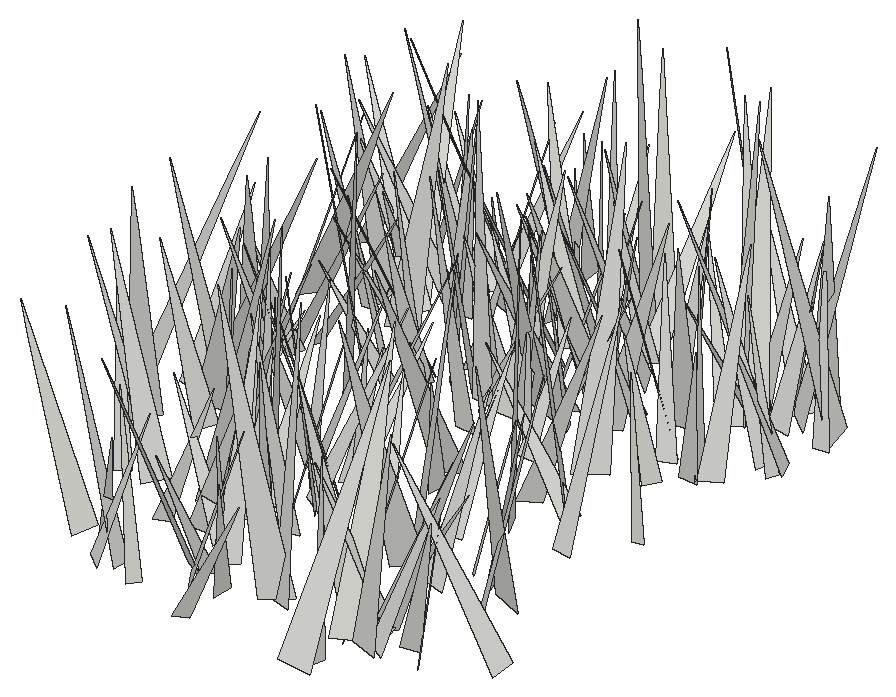
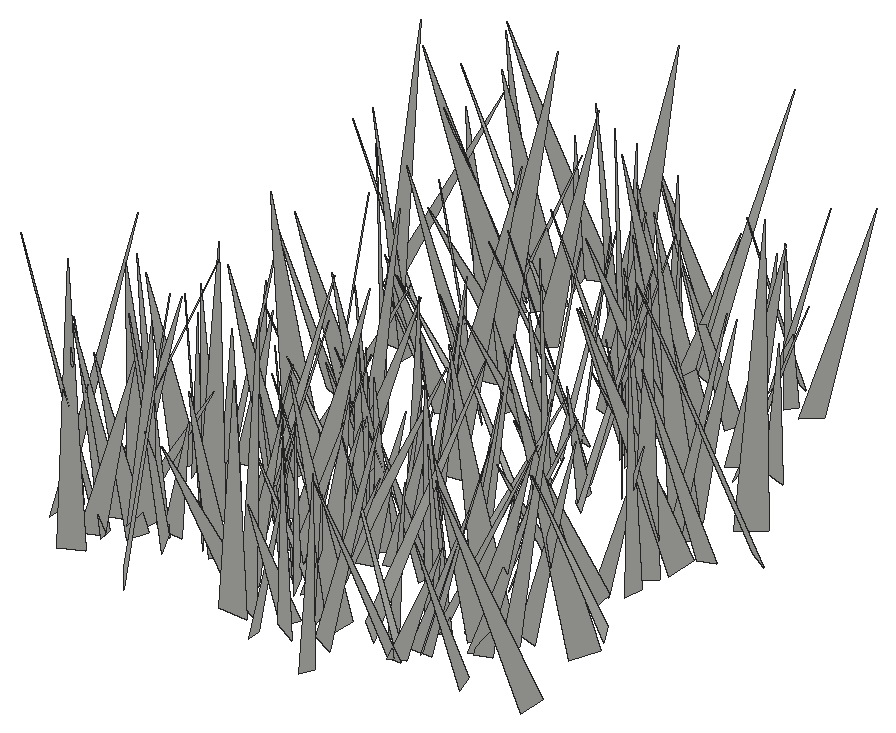
# SketchUp Ruby script. Lengths in inches.
U = 1.inch
M = Sketchup.active_model
def pt(a) = Geom::Point3d.new(a.map { |v| v * U })
def face(e, loops, mat)
  f = e.add_face(loops[0].map { |a| pt(a) })
  loops[1..].each { |l| e.add_face(l.map { |a| pt(a) }).erase! }
  f.material = f.back_material = mat if mat
  f
end
# faces: each face lists its corners as indices into pts; further lists are holes
def faces(e, pts, list, mat = nil) = list.each { |f| face(e, (f[0].is_a?(Array) ? f : [f]).map { |l| l.map { |i| pts[i] } }, mat) }
# xy, xz, yz: faces in a plane at the given z, y or x. An outline is a flat list of corners, or four numbers for a rectangle; further outlines are holes
def ring(l) = l.size == 4 ? [[l[0], l[1]], [l[2], l[1]], [l[2], l[3]], [l[0], l[3]]] : l.each_slice(2).to_a
def flat(e, list, mat, &to3) = list.each { |f| face(e, (f[0].is_a?(Array) ? f : [f]).map { |l| ring(l).map { |u, v| to3.(u, v) } }, mat) }
def xy(e, z, list, mat = nil) = flat(e, list, mat) { |x, y| [x, y, z] }
def xz(e, y, list, mat = nil) = flat(e, list, mat) { |x, z| [x, y, z] }
def yz(e, x, list, mat = nil) = flat(e, list, mat) { |y, z| [x, y, z] }
def lines(e, pts, list) = list.each { |a, b| e.add_line(pt(pts[a]), pt(pts[b])) }
# prism: a flat outline (further loops are holes) pulled along v
def prism(e, loops, v, mat = nil)
  f = face(e, loops, mat); d = Geom::Vector3d.new(v.map { |x| x * U })
  f.pushpull(f.normal.samedirection?(d) ? d.length : -d.length)
end
def box(e, o, s, mat = nil) = prism(e, [[o, [o[0] + s[0], o[1], o[2]], [o[0] + s[0], o[1] + s[1], o[2]], [o[0], o[1] + s[1], o[2]]]], [0, 0, s[2]], mat)
def at(x, y, z, deg = 0) = Geom::Transformation.translation(pt([x, y, z])) * Geom::Transformation.rotation(ORIGIN, Z_AXIS, deg.degrees)
def axes(o, x, y, z) = Geom::Transformation.new([*x, 0, *y, 0, *z, 0, *pt(o).to_a, 1])
def part(name) = M.definitions.add(name)
# library, detail: a bought-in or finely detailed component or shape, given as its bounding box
def library(name, o, s) = part(name).tap { |d| box(d.entities, o, s) }
def detail(e, o, s) = box(e.add_group.entities, o, s)
def put(e, d, t, mat = nil) = e.add_instance(d, t).tap { |i| i.material = mat if mat }
def group(e, t, mat = nil) = e.add_group.tap { |g| g.transformation = t; g.material = mat if mat }.entities
root = M.entities
c1 = part("fur_instance\#9")
p = [[0.8125,0,1.79],[0.67,-0.02,1.48],[0,-0.11,0],[0,0.11,0]]
faces(c1.entities,p,[[0,1,2,3]])
put(root,c1,axes([476.24,187.77,-21.66],[4.4489,2.71988,0.66857],[2.4928,-4.41728,1.38241],[-1.27698,0.85286,5.02786]))
put(root,c1,axes([474.66,195.15,-21.66],[5.89255,-1.31891,0.46121],[-1.38894,-5.74659,1.31223],[-0.15186,1.38261,5.89404]))
put(root,c1,axes([475.08,177.99,-21.66],[4.54632,6.46757,0.61256],[6.48609,-4.47646,-0.87508],[0.36794,-1.0028,7.85702]))
put(root,c1,axes([478.71,179.93,-21.66],[-6.26748,-0.84521,1.62615],[-0.68504,6.45447,0.7145],[1.69984,-0.51518,6.28372]))
put(root,c1,axes([476.84,179.58,-21.66],[0.12132,5.40428,1.16344],[5.42728,0.10479,-1.05269],[1.05091,-1.16504,5.30215]))
put(root,c1,axes([478.76,190.43,-21.66],[-1.01611,-5.1437,1.43202],[-5.3112,0.8243,-0.80778],[-0.54728,1.55038,5.1805]))
put(root,c1,axes([477.09,176.02,-21.66],[5.45655,-4.97036,1.37233],[-4.9464,-5.60993,-0.6508],[-1.45634,0.43117,7.35221]))
put(root,c1,axes([478.71,191.72,-21.66],[-6.33484,-0.15602,2.15214],[0.09289,6.64883,0.75543],[2.15578,-0.74496,6.29157]))
put(root,c1,axes([479.32,171.53,-21.66],[-0.14147,5.00237,0.6936],[4.87308,-0.04695,1.33257],[-1.32587,-0.70632,4.82369]))
put(root,c1,axes([477.64,183.99,-21.66],[5.74214,0.07937,1.80023],[0.34922,-5.94743,-0.85168],[-1.76782,-0.91707,5.67918]))
put(root,c1,axes([478.67,185.1,-21.66],[2.63547,-2.52355,0.88422],[-2.24578,-2.7628,-1.19134],[-1.45143,-0.30736,3.44888]))
put(root,c1,axes([480.8125,172.24,-21.66],[-5.83458,-0.97839,0.23219],[-1.00024,5.78729,-0.74851],[0.10327,0.77686,5.8685]))
put(root,c1,axes([480.66,191.54,-21.66],[-3.78677,4.88862,0.77178],[4.90876,3.58599,1.37062],[-0.63111,-1.44081,6.0299]))
put(root,c1,axes([475.72,189.9375,-21.66],[6.5822,-3.48627,0.04021],[-3.46978,-6.5418,0.80411],[0.34104,0.72931,7.40492]))
put(root,c1,axes([479.73,192.85,-21.66],[-4.18916,1.41328,1.44955],[1.84035,4.04661,1.3732],[0.84361,-1.80976,4.20247]))
put(root,c1,axes([478.39,195.45,-21.66],[4.03699,1.00135,1.00845],[0.75439,-4.0837,1.03503],[-1.2044,0.79854,4.02849]))
put(root,c1,axes([479.79,177.1,-21.66],[3.58153,-3.37168,2.12142],[-3.21603,-4.13077,-1.13573],[-2.3507,0.51427,4.78599]))
put(root,c1,axes([477.99,182.7,-21.66],[6.15158,-3.29467,0.71793],[-3.15743,-6.15236,-1.17953],[-1.18361,-0.7112,6.87789]))
put(root,c1,axes([480.25,191.67,-21.66],[-4.33285,5.33033,0.39838],[5.19442,4.31986,-1.30443],[1.26061,0.52067,6.74422]))
put(root,c1,axes([479.34,192.875,-21.66],[2.09335,-3.21544,0.11512],[-3.16402,-2.08217,-0.6229],[-0.58423,-0.24481,3.78592]))
put(root,c1,axes([477.34,180.83,-21.66],[6.84085,-1.05323,0.60817],[-1.14548,-6.7472,1.19982],[-0.40871,1.28156,6.81667]))
put(root,c1,axes([481.98,193.72,-21.66],[-6.45817,-1.9042,0.82118],[-2.02073,6.38203,-1.093],[0.4658,1.28531,6.64374]))
put(root,c1,axes([481.15,171.73,-21.66],[-4.7653,3.97573,1.88545],[4.327,4.73874,0.94381],[0.79899,-1.95123,6.13381]))
put(root,c1,axes([478.27,185.5,-21.66],[5.14686,-0.10254,0.48257],[-0.21946,-5.00543,1.27711],[-0.44184,1.29176,4.98695]))
put(root,c1,axes([481.48,166.06,-21.66],[-5.50696,2.25656,1.40845],[2.52369,5.45565,1.12666],[0.84072,-1.59571,5.84374]))
put(root,c1,axes([482.23,192.55,-21.66],[-5.87087,-0.65311,0.1721],[-0.62527,5.82501,0.77566],[0.25536,-0.75237,5.85594]))
put(root,c1,axes([481.77,194.43,-21.66],[-2.38269,3.95567,1.05235],[4.03891,2.07425,1.34786],[-0.66484,-1.57548,4.41677]))
put(root,c1,axes([482.22,195.6,-21.66],[-3.14834,2.92622,0.07201],[2.87738,3.07451,0.86494],[-0.53726,-0.68166,4.21031]))
put(root,c1,axes([478.875,186.36,-21.66],[4.0967,-0.1052,0.02727],[-0.10864,-3.93802,1.12914],[0.00278,1.12946,3.93942]))
put(root,c1,axes([482.51,186.8,-21.66],[-3.84784,-1.19504,0.32807],[-1.23606,3.62421,-1.29571],[-0.08892,1.33363,3.81512]))
put(root,c1,axes([481.8,189.2,-21.66],[-3.17916,-2.57933,0.00353],[-2.53731,3.12837,0.73174],[0.46373,-0.56605,4.02798]))
put(root,c1,axes([478.75,178.69,-21.66],[3.49272,-6.19271,0.17705],[-6.11252,-3.41157,1.25629],[1.00898,0.76914,6.99789]))
put(root,c1,axes([480.98,190.02,-21.66],[5.12672,-4.5376,2.59386],[-5.0883,-5.16347,1.02416],[-1.19461,2.5199,6.76936]))
put(root,c1,axes([482.89,191.59,-21.66],[-5.05417,-1.27819,2.14403],[-1.86511,5.15169,-1.32541],[1.65892,1.89778,5.04199]))
put(root,c1,axes([481.2,178.72,-21.66],[3.19088,3.17646,1.19509],[3.39239,-3.03309,-0.99593],[-0.09903,-1.55252,4.39087]))
put(root,c1,axes([484.76,187.57,-21.66],[-3.76268,-4.24685,0.11424],[-4.17448,3.66755,-1.15295],[-0.78896,0.84846,5.55555]))
put(root,c1,axes([484.8,164.57,-21.66],[-6.17227,-0.98801,0.5453],[-1.07692,6.06305,-1.2042],[0.3373,1.27815,6.13375]))
put(root,c1,axes([484.81,194.36,-21.66],[-4.99858,-6.00178,0.67378],[-6.03784,4.94565,-0.739],[-0.1407,0.9901,7.77567]))
put(root,c1,axes([481.07,176.93,-21.66],[1.22352,3.80068,0.33063],[3.61313,-1.04295,-1.38167],[1.22465,-0.72012,3.74608]))
put(root,c1,axes([484.16,185.24,-21.66],[-3.93279,-0.23592,0.50656],[-0.05149,3.7386,1.34138],[0.55643,-1.32147,3.70448]))
put(root,c1,axes([483.9375,176.93,-21.66],[2.37526,2.53476,1.46683],[2.25858,-2.78775,1.16004],[-1.86424,-0.14786,3.27432]))
put(root,c1,axes([482.27,192.54,-21.66],[2.19919,-5.46865,1.19281],[-5.58851,-2.07385,0.79564],[0.31218,1.39943,5.84033]))
put(root,c1,axes([482.7,183.87,-21.66],[6.58164,2.52237,2.667],[2.99732,-6.85363,-0.91486],[-2.11926,-1.85972,6.9888]))
put(root,c1,axes([485.0625,182.67,-21.66],[-5.96506,-5.04673,2.13711],[-5.35643,6.03696,-0.69462],[1.15994,1.92465,7.7826]))
put(root,c1,axes([484.43,172.75,-21.66],[-4.83197,-1.5354,1.95575],[-2.0901,4.8234,-1.3772],[1.34681,1.9768,4.87942]))
put(root,c1,axes([482.3,195.72,-21.66],[1.86244,4.7215,0.55373],[4.68693,-1.72429,-1.06173],[0.79484,-0.89561,4.96326]))
put(root,c1,axes([482.78,165.92,-21.66],[3.65052,-1.24636,0.3015],[-1.17659,-3.61738,-0.70767],[-0.50984,-0.576,3.79195]))
put(root,c1,axes([484.67,179.25,-21.66],[-4.07639,-4.57708,0.71562],[-4.52519,4.13816,0.69067],[0.99219,0.06853,6.09012]))
put(root,c1,axes([485.39,177.82,-21.66],[-6.52757,-2.25287,1.08541],[-2.07972,6.57544,1.14066],[1.38863,-0.74224,6.81054]))
put(root,c1,axes([483.55,194.23,-21.66],[-0.85908,-3.57953,0.71794],[-3.54097,0.99653,0.73143],[0.88884,0.51028,3.60778]))
put(root,c1,axes([482.57,194.99,-21.66],[4.81991,2.46867,0.79438],[2.57067,-4.76928,-0.77622],[-0.3421,-1.05666,5.35942]))
put(root,c1,axes([485.87,185.33,-21.66],[-5.27526,-0.92635,0.94955],[-1.13263,5.17215,-1.24665],[0.69057,1.40673,5.20887]))
put(root,c1,axes([484.89,178.5,-21.66],[-3.85021,0.78609,0.9669],[0.45373,3.80886,-1.28983],[1.16059,1.11875,3.71193]))
put(root,c1,axes([485.46,174.22,-21.66],[-5.53054,0.45224,1.5037],[0.10523,5.59989,-1.29715],[1.5667,1.22031,5.39525]))
put(root,c1,axes([485.76,196.62,-21.66],[-2.42816,-5.42807,1.43938],[-5.61543,2.33238,-0.67728],[-0.05217,1.5899,5.90772]))
put(root,c1,axes([486.3125,163.6,-21.66],[-4.58917,0.765,0.19448],[0.68534,4.43094,-1.25723],[0.3916,1.21042,4.47941]))
put(root,c1,axes([483.6,164.08,-21.66],[2.51167,3.62255,0.80621],[3.69421,-2.34748,-0.96099],[0.35452,-1.20325,4.30208]))
put(root,c1,axes([483.6875,169.01,-21.66],[3.11489,-2.67244,0.85057],[-2.80172,-2.90834,1.1224],[0.12545,1.40269,3.94774]))
put(root,c1,axes([483.26,173.39,-21.66],[6.3266,0.04535,0.7535],[-0.10627,-6.24313,1.26797],[-0.74735,1.27161,6.1984]))
put(root,c1,axes([485.06,186.32,-21.66],[3.85472,-3.45884,0.89823],[-3.26491,-3.94586,-1.18314],[-1.45282,-0.30973,5.04209]))
put(root,c1,axes([483.9,172.14,-21.66],[7.6269,-0.50277,1.8471],[-0.68475,-7.80192,0.70374],[-1.78765,0.84341,7.61099]))
put(root,c1,axes([484.76,199.0625,-21.66],[4.55576,-0.64185,1.19418],[-0.37344,-4.61891,-1.05794],[-1.3033,-0.92017,4.47746]))
put(root,c1,axes([487.13,169.12,-21.66],[-3.1283,2.85302,0.75954],[2.94685,2.94951,1.058],[-0.18092,-1.28978,4.09959]))
put(root,c1,axes([486.23,171.21,-21.66],[-5.56085,2.56326,1.5764],[2.25423,5.74256,-1.38556],[1.99343,0.65656,5.96435]))
put(root,c1,axes([486.22,187.08,-21.66],[4.10758,4.73433,2.04961],[4.7509,-4.49256,0.85604],[-2.01089,-0.9434,6.20913]))
put(root,c1,axes([486.87,187.87,-21.66],[-4.89402,-3.33819,1.83703],[-3.30827,5.20635,0.64726],[1.89038,0.46913,5.88863]))
put(root,c1,axes([488.79,191.91,-21.66],[-3.68425,-5.36529,0.32526],[-5.32374,3.58793,-1.11818],[-0.74155,0.8979,6.41168]))
put(root,c1,axes([486.41,173.12,-21.66],[-2.91269,3.59929,0.76549],[3.33369,2.99435,-1.39463],[1.55801,0.3218,4.41516]))
put(root,c1,axes([486.15,172.15,-21.66],[-1.6675,3.7386,1.84502],[3.94069,2.06209,-0.61692],[1.36097,-1.39013,4.04687]))
put(root,c1,axes([485.87,188.88,-21.66],[3.36091,-1.13304,0.9234],[-1.35023,-3.29337,0.87337],[-0.55977,1.1411,3.43755]))
put(root,c1,axes([487.35,194.96,-21.66],[-3.69275,-0.52533,1.17947],[-0.76187,3.77166,-0.70545],[1.04243,0.89562,3.66261]))
put(root,c1,axes([487.93,193.75,-21.66],[-0.66847,-3.61729,0.84651],[-3.58891,0.40659,-1.09666],[-0.95975,0.99906,3.51127]))
put(root,c1,axes([488.29,193.41,-21.66],[-2.02202,5.92033,1.45384],[6.05855,1.78151,1.17164],[-0.67672,-1.74024,6.14542]))
put(root,c1,axes([487.82,196.84,-21.66],[1.64216,5.46326,1.64146],[5.44457,-2.0108,1.24565],[-1.70244,-1.16093,5.56707]))
put(root,c1,axes([486.04,194.98,-21.66],[6.43486,-0.85229,1.84553],[-1.08084,-6.62327,0.70985],[-1.72168,0.97247,6.45212]))
put(root,c1,axes([486.18,173.95,-21.66],[7.03768,2.72348,2.80411],[3.28727,-7.24831,-1.21043],[-2.11523,-2.20318,7.44856]))
put(root,c1,axes([487.78,166.26,-21.66],[-3.38776,-6.42257,0.32475],[-6.36234,3.40084,0.88702],[0.93573,-0.12917,7.20691]))
put(root,c1,axes([487.82,188.95,-21.66],[1.8485,-3.49978,1.33816],[-3.45042,-2.17169,-0.91344],[-1.46071,0.70098,3.8511]))
put(root,c1,axes([485.56,169.36,-21.66],[2.4486,-4.30122,0.69777],[-4.269,-2.2075,1.37318],[0.8735,1.26866,4.75506]))
put(root,c1,axes([488.29,186.8,-21.66],[1.87849,6.8023,2.53671],[7.02619,-2.36292,1.13321],[-1.82724,-2.09291,6.96533]))
put(root,c1,axes([488.79,187.26,-21.66],[-4.99068,-1.45127,1.21381],[-1.71677,4.91279,-1.18474],[0.79513,1.49823,5.06058]))
put(root,c1,axes([488.5625,174.17,-21.66],[3.89411,3.28531,3.07479],[3.51498,-4.75969,0.63397],[-2.80935,-1.40135,5.05524]))
put(root,c1,axes([489.1,193.22,-21.66],[-4.79619,2.23097,0.90337],[2.34699,4.78153,0.65218],[0.53379,-0.97799,5.24932]))
put(root,c1,axes([488.39,166.53,-21.66],[0.67909,-3.62862,0.46379],[-3.53581,-0.77205,-0.86319],[-0.93808,0.2832,3.58928]))
put(root,c1,axes([488.13,196.03,-21.66],[-2.89622,3.26829,0.45856],[3.08153,2.89643,-1.18106],[1.18158,0.4572,4.20415]))
put(root,c1,axes([489.01,171.71,-21.66],[-0.52973,-5.32119,2.08202],[-5.65742,0.19488,-0.94137],[-0.8022,2.1395,5.26399]))
put(root,c1,axes([488.3,176.08,-21.66],[-3.60567,-4.25836,0.82426],[-4.10665,3.69659,1.13335],[1.39586,-0.12438,5.46351]))
put(root,c1,axes([485.75,181.77,-21.66],[5.05169,2.87341,0.23488],[2.86098,-4.93803,-1.1233],[0.35552,-1.09113,5.70213]))
put(root,c1,axes([488.9,189.55,-21.66],[-2.91756,2.69263,1.56889],[3.08399,2.80363,0.92331],[0.448,-1.76443,3.86133]))
put(root,c1,axes([488.51,167.69,-21.66],[-5.11212,3.73872,1.49873],[3.53116,5.32488,-1.23875],[1.93782,0.15985,6.21106]))
put(root,c1,axes([487.84,168.29,-21.66],[3.54062,0.10617,1.20258],[0.38468,-3.63127,-0.812],[-1.14433,-0.89222,3.44788]))
put(root,c1,axes([488.78,197.92,-21.66],[-4.40075,-1.21691,1.44212],[-0.98766,4.60363,0.87078],[1.60783,-0.50284,4.4821]))
put(root,c1,axes([489.28,184.29,-21.66],[1.25077,5.74635,3.18749],[6.40163,-1.79789,0.7292],[-1.48314,-2.91412,5.83551]))
put(root,c1,axes([488.14,177.04,-21.66],[-2.24113,2.46388,1.48853],[2.36542,2.65133,-0.82724],[1.6405,-0.45695,3.22631]))
put(root,c1,axes([486.77,175.98,-21.66],[4.58071,3.98416,0.78034],[4.05613,-4.44078,-1.1369],[0.17387,-1.36793,5.96354]))
put(root,c1,axes([490.03,193.15,-21.66],[-4.76219,-1.42096,1.84075],[-1.91994,4.76946,-1.2853],[1.31199,1.82182,4.80058]))
put(root,c1,axes([489.7,175.6,-21.66],[-4.04138,0.55951,1.25439],[0.25517,4.13619,-1.02282],[1.34961,0.89343,3.94964]))
put(root,c1,axes([490.82,192.64,-21.66],[-2.4507,-4.58404,1.24543],[-4.71435,2.17524,-1.27033],[-0.58261,1.68089,5.0404]))
put(root,c1,axes([490.36,196.36,-21.66],[-3.60643,-6.53276,3.39182],[-7.2869,3.70246,-0.61691],[1.0404,3.28673,7.43658]))
put(root,c1,axes([488.8,176.6,-21.66],[-0.26739,4.57604,0.32256],[4.40279,0.34673,-1.26925],[1.2883,-0.2352,4.40462]))
put(root,c1,axes([490.78,196.97,-21.66],[-0.82841,6.75025,1.93378],[7.00258,0.65031,0.72978],[-0.51887,-2.00072,6.76162]))
put(root,c1,axes([488.21,174.43,-21.66],[2.55836,5.15566,0.46861],[5.11042,-2.43162,-1.14739],[0.82709,-0.92305,5.63999]))
put(root,c1,axes([488.95,188.11,-21.66],[1.24719,-3.91493,0.4967],[-3.8954,-1.13791,0.81231],[0.63182,0.71228,4.02769]))
put(root,c1,axes([488.31,165.21,-21.66],[4.57096,2.53062,0.74602],[2.63797,-4.36083,-1.37058],[0.04077,-1.55993,5.04174]))
put(root,c1,axes([489.68,169.35,-21.66],[-1.49561,-5.63035,1.67127],[-5.71638,1.79132,0.91926],[1.34798,1.34949,5.75262]))
put(root,c1,axes([489.92,192.4,-21.66],[3.50829,2.33455,0.59392],[2.17247,-3.51961,1.00185],[-1.04078,0.52272,4.09323]))
put(root,c1,axes([489.66,170.14,-21.66],[4.69636,2.95892,0.9191],[2.85112,-4.78039,0.82137],[-1.21287,0.21986,5.48965]))
put(root,c1,axes([489.66,189.04,-21.66],[-0.19463,-4.95849,1.24268],[-5.00803,0.4343,0.94858],[1.02496,1.18047,4.8708]))
put(root,c1,axes([488.2,186.69,-21.66],[4.34126,2.62004,0.01209],[2.52851,-4.18338,-1.34808],[0.68659,-1.1602,4.88813]))
put(root,c1,axes([490.1875,188.08,-21.66],[-1.33091,-4.34516,1.37723],[-4.35803,1.6335,0.94222],[1.33595,0.99989,4.44566]))
put(root,c1,axes([491.89,190.35,-21.66],[-4.72142,-2.258,0.83052],[-2.14472,4.77905,0.80066],[1.09019,-0.37724,5.17198]))
put(root,c1,axes([491.8125,188.625,-21.66],[0.91658,-6.09487,0.23316],[-5.96683,-0.94489,-1.24341],[-1.26442,0.04079,6.03668]))
put(root,c1,axes([490.07,165.45,-21.66],[3.94789,-1.4658,0.35037],[-1.34081,-3.86465,-1.06014],[-0.68816,-0.87925,4.0756]))
put(root,c1,axes([492.36,166.5625,-21.66],[2.49125,-7.31611,3.2771],[-7.62751,-3.2193,-1.38865],[-2.46697,2.5655,7.60286]))
put(root,c1,axes([489.58,191.08,-21.66],[4.36053,2.62617,0.62372],[2.69593,-4.29581,-0.7602],[-0.13318,-0.97427,5.03319]))
put(root,c1,axes([490.16,186.51,-21.66],[-1.02594,6.32348,2.52203],[6.58274,1.57191,-1.26344],[1.73626,-2.22313,6.28034]))
put(root,c1,axes([491.23,180.76,-21.66],[2.31085,-7.14722,0.11909],[-7.10013,-2.30949,-0.83147],[-0.82765,-0.14321,7.46535]))
put(root,c1,axes([491.9375,194.39,-21.66],[1.8151,-3.86013,1.55176],[-3.9232,-2.15155,-0.76319],[-1.38458,1.03602,4.19675]))
put(root,c1,axes([490.71,192.625,-21.66],[4.61711,2.95667,1.94744],[3.35791,-4.67134,-0.86895],[-1.12198,-1.8135,5.41336]))
put(root,c1,axes([492.01,190.66,-21.66],[1.78326,-6.33726,0.7797],[-6.26284,-1.89367,-1.06754],[-1.24322,0.44943,6.49625]))
put(root,c1,axes([490.88,187.85,-21.66],[-1.24529,-7.71146,0.7872],[-7.61167,1.36728,1.35282],[1.46589,0.54863,7.69333]))
put(root,c1,axes([492.83,187.4,-21.66],[-3.64875,-2.02244,1.121],[-2.25149,3.58457,-0.86132],[0.52696,1.3118,4.08188]))
put(root,c1,axes([491.42,195.37,-21.66],[-1.51981,5.35977,0.02073],[5.22969,1.48762,-1.21441],[1.17387,0.31183,5.43711]))
put(root,c1,axes([489.99,162.49,-21.66],[3.34433,-2.45993,0.06359],[-2.39384,-3.22746,1.0454],[0.56992,0.87868,4.01783]))
put(root,c1,axes([492.64,174.16,-21.66],[-3.06168,2.49465,0.02952],[2.42804,2.99025,-0.87237],[0.57338,0.65813,3.85176]))
put(root,c1,axes([490.96,186.12,-21.66],[-2.2184,-4.85625,2.50772],[-5.03427,2.86928,1.10295],[2.1279,1.72546,5.22379]))
put(root,c1,axes([492.61,184.6875,-21.66],[1.15906,3.62365,1.13013],[3.60388,-1.42153,0.86183],[-1.19166,-0.77453,3.7056]))
put(root,c1,axes([493.05,192.97,-21.66],[-5.52274,-3.05851,1.02558],[-2.84433,5.57616,1.31266],[1.52186,-0.67738,6.17511]))
put(root,c1,axes([490.95,192.83,-21.66],[4.30698,0.82715,0.77594],[0.97071,-4.26434,-0.84231],[-0.5865,-0.98365,4.30404]))
put(root,c1,axes([492.85,166.24,-21.66],[2.9733,6.47594,2.08154],[6.51847,-3.36189,1.14821],[-1.94427,-1.36785,7.03277]))
put(root,c1,axes([491.71,179.16,-21.66],[3.65469,-1.69105,0.3912],[-1.57801,-3.61693,-0.89287],[-0.72291,-0.65395,3.92673]))
put(root,c1,axes([493.05,183.98,-21.66],[-0.85161,3.55792,0.87868],[3.50079,1.05663,-0.88551],[1.08413,-0.61714,3.54963]))
put(root,c1,axes([493.64,175.32,-21.66],[4.42049,5.15695,1.86392],[5.12768,-4.73588,0.94203],[-1.94301,-0.76574,6.72662]))
put(root,c1,axes([494.09,191.12,-21.66],[-2.87377,-5.9267,0.11201],[-5.79461,2.83495,1.33509],[1.24935,-0.48389,6.44995]))
put(root,c1,axes([495.21,168.55,-21.66],[4.87258,-2.82126,2.84071],[-2.53321,-5.63755,-1.25383],[-3.10033,0.17232,5.48903]))
put(root,c1,axes([494.65,193.14,-21.66],[3.28542,-2.52777,1.83261],[-2.97263,-3.34603,0.71392],[-0.95477,1.71946,4.08337]))
put(root,c1,axes([495.21,172.72,-21.66],[3.52334,-7.25518,1.10129],[-7.15699,-3.66725,-1.26216],[-1.62106,0.42196,7.96608]))
put(root,c1,axes([493.16,185.2,-21.66],[4.26257,2.91433,0.00484],[2.86478,-4.18851,-0.95515],[0.53516,-0.79116,5.0745]))
put(root,c1,axes([496.79,197.47,-21.66],[-6.4254,-4.61842,2.37343],[-5.01235,6.50279,-0.91585],[1.35622,2.15235,7.85982]))
put(root,c1,axes([494.95,176.11,-21.66],[-1.9043,4.31856,1.08738],[4.14528,2.15112,-1.28374],[1.62757,-0.42591,4.54184]))
put(root,c1,axes([495.16,174.45,-21.66],[3.38702,2.66566,0.2184],[2.51461,-3.29384,1.20529],[-0.91115,0.81867,4.13823]))
put(root,c1,axes([496.16,188.73,-21.66],[-3.36385,-0.86607,1.07357],[-0.51946,3.41676,1.12873],[1.27781,-0.89095,3.28504]))
put(root,c1,axes([494.32,188.43,-21.66],[4.99795,-3.82327,1.26682],[-4.01963,-4.86241,1.18375],[-0.25457,1.71502,6.18026]))
put(root,c1,axes([496.3,184.66,-21.66],[5.95771,-4.00613,4.25574],[-5.13988,-6.48421,1.09155],[-2.78246,3.40011,7.09591]))
put(root,c1,axes([497.56,192.92,-21.66],[-1.2405,4.10694,0.41743],[4.03089,1.11105,1.04764],[-0.89058,-0.69186,4.16031]))
put(root,c1,axes([496.49,178.6875,-21.66],[6.19858,3.66698,3.16063],[3.75526,-6.8827,0.6206],[-3.05522,-1.01998,7.17523]))
put(root,c1,axes([498.41,180.68,-21.66],[-4.58076,1.47717,0.18742],[1.47131,4.39705,1.30451],[-0.22897,-1.29786,4.63288]))
put(root,c1,axes([497.93,180.97,-21.66],[-5.99226,-3.56649,1.99916],[-3.93709,5.99,-1.11487],[1.10264,2.00593,6.88361]))
put(root,c1,axes([495.87,192.83,-21.66],[4.89735,3.35239,2.18214],[3.80193,-4.97328,-0.89225],[-1.24321,-2.00306,5.86741]))
put(root,c1,axes([497.58,163.13,-21.66],[-4.70779,-0.34884,1.44292],[-0.70643,4.74641,-1.15738],[1.30563,1.3103,4.57662]))
put(root,c1,axes([498.45,167.41,-21.66],[-4.68733,-0.90911,0.30449],[-0.85582,4.65242,0.7161],[0.43216,-0.64711,4.72067]))
put(root,c1,axes([497.28,165.61,-21.66],[-5.06165,5.7028,1.49455],[5.55918,5.27278,-1.292],[1.96243,-0.22764,7.51486]))
put(root,c1,axes([499.02,193.39,-21.66],[-7.08431,2.74004,0.68893],[2.60293,7.0529,-1.28499],[1.09872,0.95845,7.48626]))
put(root,c1,axes([497.29,193.79,-21.66],[-5.34624,-2.21651,3.3319],[-3.00843,5.89263,-0.90721],[2.6389,2.22728,5.71596]))
put(root,c1,axes([498.36,187.72,-21.66],[-0.93822,4.8343,1.08723],[4.93478,0.81164,0.64956],[-0.44769,-1.18472,4.88147]))
put(root,c1,axes([495.74,180.91,-21.66],[5.04993,-3.13211,0.88061],[-3.25342,-4.87587,1.31476],[-0.02926,1.58216,5.79512]))
put(root,c1,axes([497.95,188.85,-21.66],[-3.94207,-4.94022,1.13908],[-4.81769,4.09962,1.10733],[1.57897,0.1748,6.2225]))
put(root,c1,axes([498.01,173.95,-21.66],[2.52886,2.74781,0.4271],[2.47453,-2.48701,1.34889],[-1.2687,0.62635,3.48225]))
put(root,c1,axes([496.96,162.07,-21.66],[-0.59068,7.87895,1.19707],[7.83923,0.79048,-1.33468],[1.43434,-1.07565,7.78752]))
put(root,c1,axes([498.42,192.73,-21.66],[2.96295,7.07925,2.39249],[7.30087,-3.29107,0.69644],[-1.59283,-1.91622,7.64263]))
put(root,c1,axes([497.23,171.94,-21.66],[0.7475,5.23214,1.319],[5.34274,-0.53135,-0.92008],[0.75507,-1.41992,5.20456]))
put(root,c1,axes([497.0625,165.69,-21.66],[6.03648,4.13261,1.07509],[4.02235,-6.12795,0.97074],[-1.43354,0.20766,7.25088]))
put(root,c1,axes([497.01,190.76,-21.66],[1.92624,-6.27783,0.49509],[-6.26935,-1.863,0.76884],[0.59288,0.69623,6.52153]))
put(root,c1,axes([499.21,192.68,-21.66],[-5.51425,5.90533,1.65371],[5.90522,5.71303,-0.71018],[1.6541,-0.70927,8.04832]))
put(root,c1,axes([500.17,192.49,-21.66],[-1.30366,-3.70433,0.26528],[-3.50778,1.13584,-1.37745],[-1.21983,0.69265,3.67753]))
put(root,c1,axes([499.08,185.73,-21.66],[2.35364,-2.97334,1.61897],[-3.0072,-2.74184,-0.66374],[-1.55518,0.80187,3.73361]))
put(root,c1,axes([497.02,169.23,-21.66],[3.6219,-1.04912,0.12415],[-1.02885,-3.40219,1.26523],[0.23987,1.24847,3.55218]))
put(root,c1,axes([500.51,195.17,-21.66],[-3.89894,3.87426,1.21258],[4.05705,3.77806,0.97396],[0.14352,-1.54866,5.40953]))
put(root,c1,axes([498.74,194.01,-21.66],[4.04203,-2.33275,1.48439],[-2.65208,-4.01454,0.91276],[-0.78205,1.55722,4.57675]))
put(root,c1,axes([500.52,187.47,-21.66],[-4.80095,-0.85986,1.55653],[-1.24807,4.82151,-1.18603],[1.26668,1.49164,4.73094]))
put(root,c1,axes([498.43,165.32,-21.66],[1.5633,5.69815,3.01797],[6.40687,-1.02237,-1.38843],[0.72737,-3.24142,5.74326]))
put(root,c1,axes([499.92,178.03,-21.66],[1.80185,5.93958,0.37976],[5.89361,-1.83593,0.75111],[-0.82954,-0.14229,6.16126]))
put(root,c1,axes([498.9,165.66,-21.66],[2.45412,4.72767,0.6627],[4.74881,-2.3413,-0.8831],[0.48874,-0.99004,5.25297]))
put(root,c1,axes([503.08,190.53,-21.66],[-6.30191,-3.29477,0.26908],[-3.30318,6.25333,-0.79169],[-0.13009,0.82599,7.06702]))
put(root,c1,axes([498.08,167.3125,-21.66],[6.2285,-2.9564,0.62521],[-3.02175,-6.08711,1.31964],[0.01382,1.46019,6.76705]))
put(root,c1,axes([502.11,190.39,-21.66],[-4.9541,1.83691,1.27432],[2.05779,4.95762,0.85363],[0.87385,-1.26054,5.21428]))
put(root,c1,axes([500.17,186.98,-21.66],[0.87128,-4.23502,0.75689],[-4.24446,-0.72019,0.85631],[0.702,0.90186,4.23807]))
put(root,c1,axes([501.09,187.53,-21.66],[-4.2045,3.84796,1.64776],[3.68267,4.51063,-1.13666],[1.98995,-0.21727,5.58504]))
put(root,c1,axes([499.51,173.27,-21.66],[5.83398,1.13984,1.03884],[1.35175,-5.73614,-1.2974],[-0.74243,-1.48703,5.80098]))
put(root,c1,axes([502.08,180.97,-21.66],[0.5553,3.90242,1.15183],[3.90207,-0.84018,0.96535],[-1.15302,-0.96393,3.8217]))
put(root,c1,axes([500,194.82,-21.66],[5.07227,1.20948,1.05659],[1.39553,-5.05165,-0.91676],[-0.7948,-1.15114,5.13326]))
put(root,c1,axes([500.46,193.26,-21.66],[0.08637,4.97569,1.67082],[5.15736,0.22998,-0.95146],[0.97504,-1.65717,4.88463]))
put(root,c1,axes([501.4,165.65,-21.66],[-2.88957,-1.62735,2.00469],[-2.2228,3.09866,-0.68855],[1.31385,1.66334,3.24403]))
put(root,c1,axes([500.14,166.68,-21.66],[2.04033,-4.0488,0.48109],[-4.03745,-1.93127,0.8697],[0.56854,0.81522,4.44965]))
put(root,c1,axes([502.98,189.71,-21.66],[-4.26519,0.30143,0.24037],[0.24291,4.17451,-0.92459],[0.29939,0.9072,4.17466]))
put(root,c1,axes([500.9,172.8,-21.66],[-1.7083,-7.51191,1.45388],[-7.48357,1.95063,1.28533],[1.59333,1.10775,7.59572]))
put(root,c1,axes([503.07,194.4,-21.66],[-7.82049,-1.65264,1.82204],[-1.48703,8.01344,0.88582],[1.95953,-0.51451,7.94397]))
put(root,c1,axes([500.36,196.86,-21.66],[1.17808,-6.7396,1.1437],[-6.76699,-0.98532,1.16408],[0.96855,1.31342,6.74203]))
put(root,c1,axes([501.4,169.96,-21.66],[4.49985,4.45709,1.03745],[4.28289,-4.6143,1.2473],[-1.61209,0.1822,6.20956]))
put(root,c1,axes([504.62,167.83,-21.66],[-6.1435,0.43905,0.01492],[0.43419,6.03663,1.1429],[-0.06685,-1.14104,6.05221]))
put(root,c1,axes([500.69,194.43,-21.66],[4.61104,6.12434,1.67223],[6.3457,-4.50796,-0.9879],[-0.18966,-1.93296,7.60219]))
put(root,c1,axes([503.1875,193.02,-21.66],[0.59003,4.76484,1.13067],[4.77949,-0.80843,0.91275],[-1.06703,-0.9864,4.71367]))
